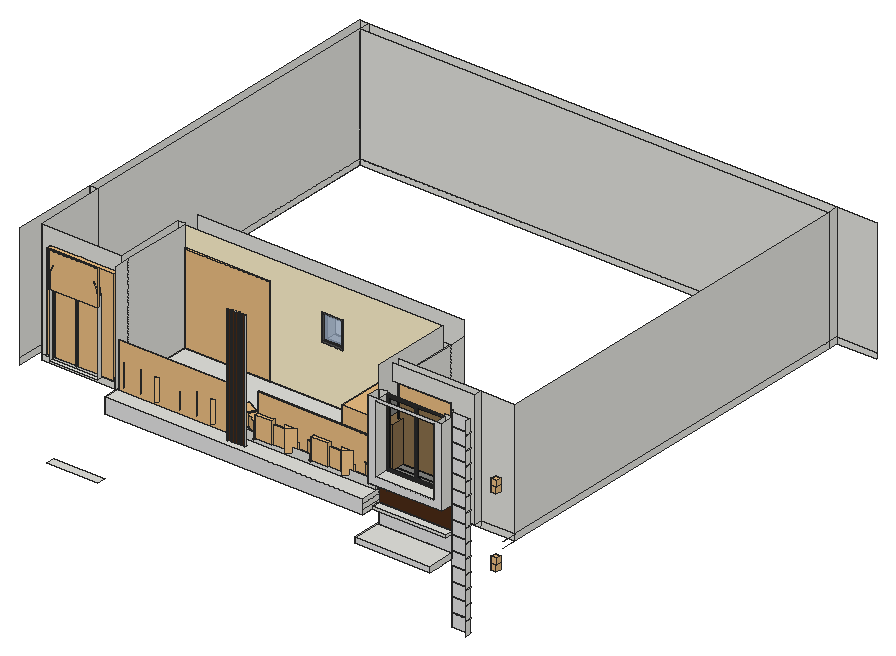
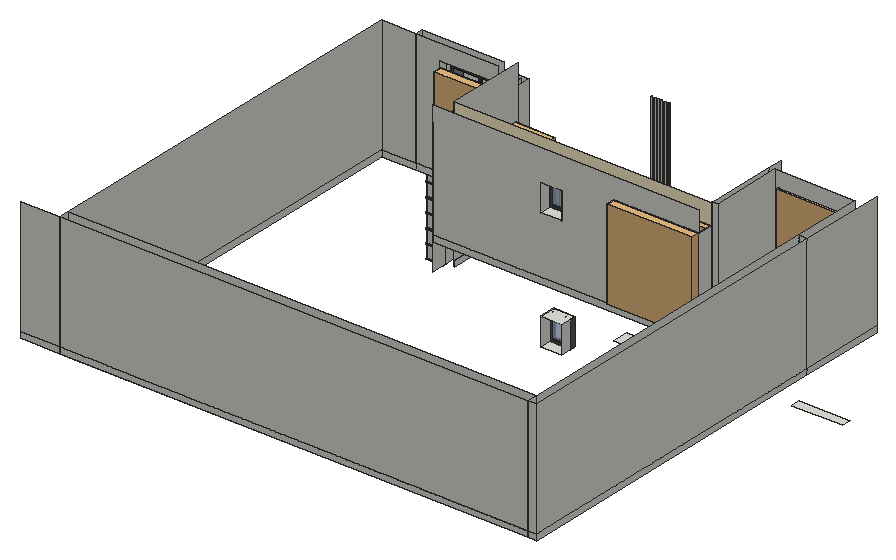
# SketchUp Ruby script. Lengths in inches.
U = 1.inch
M = Sketchup.active_model
def pt(a) = Geom::Point3d.new(a.map { |v| v * U })
def face(e, loops, mat)
  f = e.add_face(loops[0].map { |a| pt(a) })
  loops[1..].each { |l| e.add_face(l.map { |a| pt(a) }).erase! }
  f.material = f.back_material = mat if mat
  f
end
# faces: each face lists its corners as indices into pts; further lists are holes
def faces(e, pts, list, mat = nil) = list.each { |f| face(e, (f[0].is_a?(Array) ? f : [f]).map { |l| l.map { |i| pts[i] } }, mat) }
# xy, xz, yz: faces in a plane at the given z, y or x. An outline is a flat list of corners, or four numbers for a rectangle; further outlines are holes
def ring(l) = l.size == 4 ? [[l[0], l[1]], [l[2], l[1]], [l[2], l[3]], [l[0], l[3]]] : l.each_slice(2).to_a
def flat(e, list, mat, &to3) = list.each { |f| face(e, (f[0].is_a?(Array) ? f : [f]).map { |l| ring(l).map { |u, v| to3.(u, v) } }, mat) }
def xy(e, z, list, mat = nil) = flat(e, list, mat) { |x, y| [x, y, z] }
def xz(e, y, list, mat = nil) = flat(e, list, mat) { |x, z| [x, y, z] }
def yz(e, x, list, mat = nil) = flat(e, list, mat) { |y, z| [x, y, z] }
def lines(e, pts, list) = list.each { |a, b| e.add_line(pt(pts[a]), pt(pts[b])) }
# prism: a flat outline (further loops are holes) pulled along v
def prism(e, loops, v, mat = nil)
  f = face(e, loops, mat); d = Geom::Vector3d.new(v.map { |x| x * U })
  f.pushpull(f.normal.samedirection?(d) ? d.length : -d.length)
end
def box(e, o, s, mat = nil) = prism(e, [[o, [o[0] + s[0], o[1], o[2]], [o[0] + s[0], o[1] + s[1], o[2]], [o[0], o[1] + s[1], o[2]]]], [0, 0, s[2]], mat)
def at(x, y, z, deg = 0) = Geom::Transformation.translation(pt([x, y, z])) * Geom::Transformation.rotation(ORIGIN, Z_AXIS, deg.degrees)
def axes(o, x, y, z) = Geom::Transformation.new([*x, 0, *y, 0, *z, 0, *pt(o).to_a, 1])
def part(name) = M.definitions.add(name)
# library, detail: a bought-in or finely detailed component or shape, given as its bounding box
def library(name, o, s) = part(name).tap { |d| box(d.entities, o, s) }
def detail(e, o, s) = box(e.add_group.entities, o, s)
def put(e, d, t, mat = nil) = e.add_instance(d, t).tap { |i| i.material = mat if mat }
def group(e, t, mat = nil) = e.add_group.tap { |g| g.transformation = t; g.material = mat if mat }.entities
root = M.entities
M.materials.add("Glass_Tinted_Gray").color = [0, 0, 0]
M.materials["Glass_Tinted_Gray"].alpha = 0.125
M.materials.add("Material__1").color = [95, 70, 46]
M.materials.add("[0135_DarkGray]").color = [81, 81, 81]
M.materials.add("[Color D01]").color = [255, 242, 204]
M.materials.add("[Color M01]").color = [226, 226, 226]
M.materials.add("[Color_006]").color = [86, 86, 86]
M.materials.add("[Mirror 02]").color = [229, 229, 229]
M.materials.add("[Terrazzo Light Blue]").color = [196, 214, 227]
M.materials.add("[Translucent Glass Gray]").color = [128, 128, 128]
M.materials["[Translucent Glass Gray]"].alpha = 0.5
M.materials.add("[Translucent_Glass_Gray]1").color = [167, 187, 214]
M.materials["[Translucent_Glass_Gray]1"].alpha = 0.8
M.materials.add("[Wood Veneer 01]").color = [76, 44, 23]
c1 = part("BIC_Bike Shop - Window - Small")
xy(c1.entities,-8,[[[0,0,36,36],[2,2,34,34]]],"[Color_006]")
xy(c1.entities,-4,[[2,2,34,34]],"[Translucent_Glass_Gray]1")
xy(c1.entities,0,[[[0,0,36,36],[2,2,34,34]]],"[Color_006]")
xz(c1.entities,0,[[0,-8,36,0]],"[Color_006]")
xz(c1.entities,2,[[2,-8,34,-4],[2,-4,34,0]],"[Color_006]")
xz(c1.entities,34,[[2,-8,34,-4],[2,-4,34,0]],"[Color_006]")
xz(c1.entities,36,[[0,-8,36,0]],"[Color_006]")
yz(c1.entities,0,[[0,-8,36,0]],"[Color_006]")
yz(c1.entities,2,[[2,-8,34,-4],[2,-4,34,0]],"[Color_006]")
yz(c1.entities,34,[[2,-8,34,-4],[2,-4,34,0]],"[Color_006]")
yz(c1.entities,36,[[0,-8,36,0]],"[Color_006]")
c2 = library("SPOT",[0,0,1.68],[5.4375,5.4375,6.28])
c3 = part("Group\#3")
xy(c3.entities,0,[[0,0,32.48,1.97]])
xy(c3.entities,0.98,[[0.98,0,31.5,0.98],[0.98,0.98,31.5,1.97]])
xy(c3.entities,8.86,[[0.98,0,31.5,0.98],[0.98,0.98,31.5,1.97]])
xy(c3.entities,9.84,[[0,0,32.48,1.97]])
xz(c3.entities,0,[[[0,0,32.48,9.84],[0.98,0.98,31.5,8.86]]])
xz(c3.entities,0.98,[[0.98,0.98,31.5,8.86]],"[Translucent Glass Gray]")
xz(c3.entities,1.97,[[[0,0,32.48,9.84],[0.98,0.98,31.5,8.86]]])
yz(c3.entities,0,[[0,0,1.97,9.84]])
yz(c3.entities,0.98,[[0,0.98,0.98,8.86],[0.98,0.98,1.97,8.86]])
yz(c3.entities,31.5,[[0,0.98,0.98,8.86],[0.98,0.98,1.97,8.86]])
yz(c3.entities,32.48,[[0,0,1.97,9.84]])
c4 = part("Group\#4")
xy(c4.entities,0,[[0,0,32.48,1.97]])
xy(c4.entities,0.98,[[0.98,0,31.5,0.98],[0.98,0.98,31.5,1.97]])
xy(c4.entities,71.85,[[0.98,0,31.5,0.98],[0.98,0.98,31.5,1.97]])
xy(c4.entities,72.83,[[0,0,32.48,1.97]])
xz(c4.entities,0,[[[0,0,32.48,72.83],[0.98,0.98,31.5,71.85]]])
xz(c4.entities,0.98,[[0.98,0.98,31.5,71.85]],"[Translucent Glass Gray]")
xz(c4.entities,1.97,[[[0,0,32.48,72.83],[0.98,0.98,31.5,71.85]]])
yz(c4.entities,0,[[0,0,1.97,72.83]])
yz(c4.entities,0.98,[[0,0.98,0.98,71.85],[0.98,0.98,1.97,71.85]])
yz(c4.entities,31.5,[[0,0.98,0.98,71.85],[0.98,0.98,1.97,71.85]])
yz(c4.entities,32.48,[[0,0,1.97,72.83]])
c5 = part("FIXED+GLASS+WINDOW+WITH+TRANSOM")
g1 = group(c5.entities,at(0,0,0))
xy(g1,0,[[0,0,70.86,3.9375]])
xy(g1,1.97,[[1.97,0,34.45,0.98],[36.42,0,68.9,3.9375],[1.97,2.95,34.45,3.9375]])
xy(g1,86.61,[[1.97,0,34.45,3.9375],[34.45,0,36.42,3.9375],[36.42,0,68.9,3.9375]])
xy(g1,88.58,[[0,0,70.86,3.9375]])
xz(g1,0,[[[0,0,70.86,88.58],[1.97,1.97,34.45,86.61],[36.42,1.97,68.9,86.61]]])
xz(g1,3.9375,[[[0,0,70.86,88.58],[1.97,1.97,34.45,86.61],[36.42,1.97,68.9,86.61]]])
yz(g1,0,[[0,0,3.9375,88.58]])
yz(g1,1.97,[[0,1.97,3.9375,74.8],[0,76.77,3.9375,86.61]])
yz(g1,34.45,[[0,1.97,3.9375,86.61]])
yz(g1,36.42,[[0,1.97,3.9375,86.61]])
yz(g1,68.9,[[0,1.97,3.9375,86.61]])
yz(g1,70.86,[[0,0,3.9375,88.58]])
g2 = group(g1,at(1.97,0,74.8))
box(g2,[0,0,0],[66.93,3.9375,1.97])
put(g1,c3,at(1.97,0.98,76.77))
put(g1,c3,at(36.42,0.98,76.77))
put(g1,c4,at(1.97,0.98,1.97))
put(g1,c4,at(36.42,0.98,1.97))
c6 = library("Sliding Door",[0,0,0],[94.49,5.83,91.73])
c7 = library("Flora+17",[-57.52,158.6,-38.64],[66.99,62.88,77.28])
c8 = part("glass-railing")
detail(c8.entities,[0,0,0],[1.26,75.59,33.1875])
c9 = library("Areca palm plant",[0,0,0],[49.1,36.6,54.46])
c10 = library("Group20\#1",[-20.81,-17.08,3.79],[39.86,39.43,37.51])
c11 = library("Group\#74",[-84.69,-90.07,-0.36],[176.51,175.13,171.4])
c12 = library("Group\#130",[-7.34,-1.2,0],[38.67,35.81,49.04])
c13 = library("Group38\#2",[14.01,28.44,-23.43],[18.58,18.32,38.89])
c14 = part("Group\#11")
put(c14.entities,c9,axes([-6.2,56.6,6.08],[0.45017,-0.56191,0],[0.66137,0.52986,0],[0,0,0.72]))
put(c14.entities,c9,axes([-6.2,158.41,6.08],[0.45017,-0.56191,0],[0.66137,0.52986,0],[0,0,0.72]))
put(c14.entities,c10,axes([18.97,181.79,4.77],[0,0.85,0],[-0.85,0,0],[0,0,0.85]))
put(c14.entities,c11,axes([14.93,71.3,6.05],[-0.04961,-0.08593,0],[0.08593,-0.04961,0],[0,0,0.10522]))
put(c14.entities,c11,axes([14.93,91.37,6.05],[-0.04961,-0.08593,0],[0.08593,-0.04961,0],[0,0,0.10522]))
put(c14.entities,c10,axes([18.97,79.98,4.77],[0,0.85,0],[-0.85,0,0],[0,0,0.85]))
put(c14.entities,c12,axes([24.9375,191.72,8],[0,0.79,0],[-0.79,0,0],[0,0,0.79]))
put(c14.entities,c11,axes([17.19,223.04,6.07],[-0.08133,-0.14087,0],[0.14087,-0.08133,0],[0,0,0.1725]))
put(c14.entities,c12,axes([24.9375,89.91,8],[0,0.79,0],[-0.79,0,0],[0,0,0.79]))
put(c14.entities,c11,axes([14.93,44.05,6.05],[-0.04961,-0.08593,0],[0.08593,-0.04961,0],[0,0,0.10522]))
put(c14.entities,c11,axes([14.93,145.87,6.05],[-0.04961,-0.08593,0],[0.08593,-0.04961,0],[0,0,0.10522]))
put(c14.entities,c13,axes([-4.1,100.66,28.17],[0.8848,0,0],[0,0.94674,0],[0,0,0.85826]))
put(c14.entities,c11,axes([14.93,173.12,6.05],[-0.04961,-0.08593,0],[0.08593,-0.04961,0],[0,0,0.10522]))
put(c14.entities,c13,axes([-4.1,-1.15,28.17],[0.8848,0,0],[0,0.94674,0],[0,0,0.85826]))
put(c14.entities,c11,axes([17.19,121.23,6.07],[-0.08133,-0.14087,0],[0.14087,-0.08133,0],[0,0,0.1725]))
put(c14.entities,c11,axes([14.93,193.18,6.05],[-0.04961,-0.08593,0],[0.08593,-0.04961,0],[0,0,0.10522]))
put(c14.entities,c11,axes([17.19,15.79,6.07],[-0.08133,-0.14087,0],[0.14087,-0.08133,0],[0,0,0.1725]))
g3 = group(c14.entities,at(0,0,0))
xy(g3,0,[[0,0,6,234.8],[30,0,36,234.8]])
xy(g3,3,[[6,0,30,234.8]])
xy(g3,7,[[6,5,30,229.8]],"Material__1")
xy(g3,15,[[[0,0,36,234.8],[6,5,30,229.8]]])
xz(g3,0,[[0,0,6,0,6,3,30,3,30,0,36,0,36,15,0,15]])
xz(g3,5,[[6,7,30,15]])
xz(g3,229.8,[[6,7,30,15]])
xz(g3,234.8,[[0,0,0,15,36,15,36,0,30,0,30,3,6,3,6,0]])
yz(g3,0,[[0,0,234.8,15]])
yz(g3,6,[[0,0,234.8,3],[5,7,229.8,15]])
yz(g3,30,[[0,0,234.8,3],[5,7,229.8,15]])
yz(g3,36,[[0,0,234.8,15]])
c15 = library("Curtains",[0,0,0],[121.73,8.19,117.22])
c16 = part("PENTEK_RP Fineline 50S_Sliding_DoorCase_E1")
box(c16.entities,[0,0,0],[1.51,3.66,99.27],"[0135_DarkGray]")
c17 = part("PENTEK_RP Fineline 50S_SlidingDooe_Case_E2")
box(c17.entities,[0,0,0],[96.25,3.66,1.51],"[0135_DarkGray]")
c18 = part("pentek_RP Fineline 50S_SlidingDoor_Case")
put(c18.entities,c16,at(97.76,0,0))
put(c18.entities,c17,at(1.51,0,0))
put(c18.entities,c16,at(0,0,0))
put(c18.entities,c17,at(1.51,0,97.76))
c19 = part("PENTEK_RP Fineline 50S_SlidingDoor_GlazingBead_2")
box(c19.entities,[0,0,0],[0.56,0.59,94.39],"[0135_DarkGray]")
c20 = part("PENTEK_RP Fineline 50S_SlidingDoor_Glass")
box(c20.entities,[0,0,0],[46.58,0.16,94.39],"Glass_Tinted_Gray")
c21 = part("PENTEK_RP Fineline 50S_SlidingDoor_GlazingBead")
box(c21.entities,[0,0,0],[45.47,0.59,0.56],"[0135_DarkGray]")
c22 = part("PENTEK_RP Fineline 50S_SlidingDoor_Leaf_E1")
xy(c22.entities,0,[[0,0,0.93,1.97],[0.93,1.57,1.49,1.97]],"[0135_DarkGray]")
xy(c22.entities,96.25,[[0,0,0.93,0,0.93,1.57,1.49,1.57,1.49,1.97,0,1.97]],"[0135_DarkGray]")
xz(c22.entities,0,[[0,0,0.93,96.25]],"[0135_DarkGray]")
xz(c22.entities,1.57,[[0.93,0,1.49,95.32],[0.93,95.32,1.49,96.25]],"[0135_DarkGray]")
xz(c22.entities,1.97,[[0,0,1.49,96.25]],"[0135_DarkGray]")
yz(c22.entities,0,[[0,0,1.97,96.25]],"[0135_DarkGray]")
yz(c22.entities,0.93,[[0,0,1.57,0.93],[0,0.93,1.57,95.32],[0,95.32,1.57,96.25]],"[0135_DarkGray]")
yz(c22.entities,1.49,[[1.57,0,1.97,95.32],[1.57,95.32,1.97,96.25]],"[0135_DarkGray]")
c23 = part("PENTEK_RP Fineline 50S_SlidingDoor_Leaf_E2")
xy(c23.entities,0,[[0,0,0,1.57,0.56,1.57,0.56,1.97,46.02,1.97,46.02,1.57,46.58,1.57,46.58,0]],"[0135_DarkGray]")
xy(c23.entities,0.93,[[0,0,46.58,1.57]],"[0135_DarkGray]")
xy(c23.entities,1.49,[[0.56,1.57,46.02,1.97]],"[0135_DarkGray]")
xz(c23.entities,0,[[0,0,46.58,0.93]],"[0135_DarkGray]")
xz(c23.entities,1.57,[[0,0,0.56,0.93],[46.02,0,46.58,0.93],[0.56,0.93,46.02,1.49]],"[0135_DarkGray]")
xz(c23.entities,1.97,[[0.56,0,46.02,1.49]],"[0135_DarkGray]")
yz(c23.entities,0,[[0,0,1.57,0.93]],"[0135_DarkGray]")
yz(c23.entities,0.56,[[1.57,0,1.97,0.93],[1.57,0.93,1.97,1.49]],"[0135_DarkGray]")
yz(c23.entities,46.02,[[1.57,0,1.97,0.93],[1.57,0.93,1.97,1.49]],"[0135_DarkGray]")
yz(c23.entities,46.58,[[0,0,1.57,0.93]],"[0135_DarkGray]")
c24 = part("PENTEK_RP Fineline S_SlidingDoor_Leaf1")
put(c24.entities,c19,at(0.93,0,0.93))
put(c24.entities,c19,at(46.96,0,0.93))
put(c24.entities,c20,at(1.49,1.42,0.93))
put(c24.entities,c21,at(1.49,0,0.93))
put(c24.entities,c20,at(1.49,0.59,0.93),"[Terrazzo Light Blue]")
put(c24.entities,c22,at(0,0,0))
put(c24.entities,c22,axes([48.44,0,0],[-1,0,0],[0,1,0],[0,0,1]))
put(c24.entities,c23,axes([0.93,0,96.25],[1,0,0],[0,1,0],[0,0,-1]))
put(c24.entities,c23,at(0.93,0,0))
put(c24.entities,c21,at(1.49,0,94.77))
c25 = part("PENTEK_RP Fineline 50S_SlidingDoor_Leaf2")
put(c25.entities,c20,at(1.49,1.42,0.93))
put(c25.entities,c21,at(1.49,0,94.77))
put(c25.entities,c19,at(46.96,0,0.93))
put(c25.entities,c20,at(1.49,0.59,0.93),"[Mirror 02]")
put(c25.entities,c19,at(0.93,0,0.93))
put(c25.entities,c22,at(0,0,0))
put(c25.entities,c22,axes([48.44,0,0],[-1,0,0],[0,1,0],[0,0,1]))
put(c25.entities,c21,at(1.49,0,0.93))
put(c25.entities,c23,axes([0.93,0,96.25],[1,0,0],[0,1,0],[0,0,-1]))
put(c25.entities,c23,at(0.93,0,0))
c26 = part("PENTEK - Slimmest Steel Sliding Door / Window\#1")
put(c26.entities,c18,at(0,-1.88,-0.09))
put(c26.entities,c24,at(1.51,-2.27,1.42))
put(c26.entities,c25,at(49.32,-0.3,1.42))
c27 = library("Group\#1",[0,0,0],[33.46,1.57,19.69])
xy(root,167.92,[[733.09,261.68,751.93,263.24]])
xy(root,171.49,[[314.4,263.24,366.4,272.46]])
xy(root,181.28,[[733.09,261.68,751.93,263.24]])
xy(root,182.22,[[733.09,261.68,751.93,263.24]])
xy(root,195.58,[[733.09,261.68,751.93,263.24]])
xy(root,196.52,[[733.09,261.68,751.93,263.24]])
xy(root,199.5625,[[531.79,345.71,553.72,362.65]])
xy(root,209.875,[[733.09,261.68,751.93,263.24]])
xy(root,210.8125,[[733.09,261.68,751.93,263.24]])
xy(root,224.18,[[733.09,261.68,751.93,263.24]])
xy(root,225.11,[[733.09,261.68,751.93,263.24]])
xy(root,227.9375,[[531.79,345.71,553.72,362.65]])
xy(root,229.87,[[664.71,249.36,724.59,279.2],[664.71,279.2,665.11,345.71],[665.11,279.2,665.59,345.71]])
xy(root,229.99,[[[655.52,234.3,732.65,249.36],[693.1875,238.33,693.82,238.42,694.41,238.66,694.91,239.05,695.3,239.55,695.54,240.14,695.625,240.77,695.54,241.4,695.3,241.99,694.91,242.49,694.41,242.88,693.82,243.125,693.1875,243.21,692.56,243.125,691.97,242.88,691.46,242.49,691.08,241.99,690.83,241.4,690.75,240.77,690.83,240.14,691.08,239.55,691.46,239.05,691.97,238.66,692.56,238.42]]])
xy(root,230.43,[[655.52,249.36,657.09,345.71],[657.09,249.36,732.65,263.24],[732.65,249.36,733.09,263.24]])
xy(root,230.62,[[693.1875,238.33,692.56,238.42,691.97,238.66,691.46,239.05,691.08,239.55,690.83,240.14,690.75,240.77,690.83,241.4,691.08,241.99,691.46,242.49,691.97,242.88,692.56,243.125,693.1875,243.21,693.82,243.125,694.41,242.88,694.91,242.49,695.3,241.99,695.54,241.4,695.625,240.77,695.54,240.14,695.3,239.55,694.91,239.05,694.41,238.66,693.82,238.42]])
xy(root,231.125,[[390.34,345.71,390.9,362.65],[390.9,345.71,478.4,362.65]])
xy(root,235.64,[[655.52,234.3,732.65,234.3,732.65,263.24,657.09,263.24,657.09,345.71,655.52,345.71]])
xy(root,238.47,[[733.09,261.68,751.93,263.24]])
xy(root,239.41,[[733.09,261.68,751.93,263.24]])
xy(root,252.77,[[733.09,261.68,751.93,263.24]])
xy(root,253.375,[[657.09,254.43,733.09,263.24]])
xy(root,253.375,[[[390.34,242.18,657.09,345.71],[447.91,289.875,449.21,289.96,450.45,290.37,451.53,291.09,452.4,292.07,452.98,293.24,453.24,294.52,453.16,295.82,452.75,297.06,452.03,298.14,451.05,299.01,449.88,299.59,448.6,299.85,447.3,299.77,446.0625,299.36,444.97,298.64,444.11,297.66,443.53,296.49,443.27,295.21,443.35,293.91,443.76,292.67,444.48,291.58,445.46,290.72,446.625,290.14],[595.53,289.875,596.83,289.96,598.07,290.37,599.16,291.09,600.02,292.07,600.61,293.24,600.87,294.52,600.79,295.82,600.37,297.06,599.65,298.14,598.67,299.01,597.51,299.59,596.23,299.85,594.92,299.77,593.6875,299.36,592.6,298.64,591.73,297.66,591.15,296.49,590.89,295.21,590.97,293.91,591.39,292.67,592.11,291.58,593.08,290.72,594.25,290.14]]],"[Wood Veneer 01]")
xy(root,253.71,[[733.09,261.68,751.93,263.24]])
xy(root,254.4375,[[447.91,289.875,446.625,290.14,445.46,290.72,444.48,291.58,443.76,292.67,443.35,293.91,443.27,295.21,443.53,296.49,444.11,297.66,444.97,298.64,446.0625,299.36,447.3,299.77,448.6,299.85,449.88,299.59,451.05,299.01,452.03,298.14,452.75,297.06,453.16,295.82,453.24,294.52,452.98,293.24,452.4,292.07,451.53,291.09,450.45,290.37,449.21,289.96],[595.53,289.875,594.25,290.14,593.08,290.72,592.11,291.58,591.39,292.67,590.97,293.91,590.89,295.21,591.15,296.49,591.73,297.66,592.6,298.64,593.6875,299.36,594.92,299.77,596.23,299.85,597.51,299.59,598.67,299.01,599.65,298.14,600.37,297.06,600.79,295.82,600.87,294.52,600.61,293.24,600.02,292.07,599.16,291.09,598.07,290.37,596.83,289.96]])
xy(root,255.91,[[657.09,254.43,733.09,263.24]])
xy(root,258,[[292.06,345.71,301.28,694.43],[301.28,683.75,784.56,694.43]])
xy(root,259.25,[[511.65,248.63,512.53,250.63],[529.78,248.63,530.65,250.63],[526.41,249.32,529.24,250.63],[512.53,249.76,515.36,250.63],[516,249.76,518.83,250.63],
  [519.47,249.76,522.3,250.63],[522.9375,249.76,525.77,250.63]])
xy(root,264,[[665.11,271.58,749.59,279.2],[292.06,345.71,301.28,694.43],[301.28,683.75,784.56,694.43]])
xy(root,267.07,[[733.09,261.68,751.93,263.24]])
xy(root,267.28,[[316.75,263.24,366.25,272.46]])
xy(root,268.01,[[733.09,261.68,751.93,263.24]])
xy(root,268.625,[[390.34,242.18,657.09,345.71],[511.65,248.63,512.53,250.63],[529.78,248.63,530.65,250.63],[512.53,249.32,515.36,250.63],[516,249.32,518.83,250.63],
  [519.47,249.32,522.3,250.63],[522.9375,249.32,525.77,250.63],[526.41,249.32,529.24,250.63],[390.34,345.71,390.9,362.65],[390.9,345.71,478.4,362.65]])
xy(root,280.21,[[657.09,249.36,732.9,263.24]])
xy(root,281.37,[[733.09,261.68,751.93,263.24]])
xy(root,282.31,[[733.09,261.68,751.93,263.24]])
xy(root,288.24,[[664.71,249.36,724.59,263.24],[664.71,263.24,724.59,263.24,724.59,271.58,665.11,271.58,665.11,279.2,664.71,279.2],[665.11,271.58,724.59,279.2]])
xy(root,292.81,[[664.05,279.2,665.11,345.71]])
xy(root,295.67,[[733.09,261.68,751.93,263.24]])
xy(root,296.61,[[733.09,261.68,751.93,263.24]])
xy(root,309.97,[[733.09,261.68,751.93,263.24]])
xy(root,310.91,[[733.09,261.68,751.93,263.24]])
xy(root,323.625,[[531.79,345.71,553.72,362.65]])
xy(root,324.27,[[733.09,261.68,751.93,263.24]])
xy(root,325.2,[[733.09,261.68,751.93,263.24]])
xy(root,338.57,[[733.09,261.68,751.93,263.24]])
xy(root,339.5,[[733.09,261.68,751.93,263.24]])
xy(root,352,[[531.79,345.71,553.72,362.65]])
xy(root,352.86,[[733.09,261.68,751.93,263.24]])
xy(root,353.8,[[733.09,261.68,751.93,263.24]])
xz(root,234.3,[[655.52,229.99,732.65,235.64]],"[Color M01]")
xz(root,242.18,[[390.34,253.375,657.09,268.625]],"[Color M01]")
xz(root,248.63,[[511.65,268.625,512.53,389.875],[529.78,268.625,530.65,389.875]])
xz(root,249.32,[[512.53,268.625,515.36,389.875],[516,268.625,518.83,389.875],[519.47,268.625,522.3,389.875],[522.9375,268.625,525.77,389.875],[526.41,268.625,529.24,389.875]],"[Wood Veneer 01]")
xz(root,249.36,[[655.52,229.99,657.09,230.43],[657.09,229.99,732.65,230.43]])
xz(root,249.36,[[[657.09,280.21,732.9,361.12],[664.71,288.24,724.59,358.37]]],"[Color M01]")
xz(root,254.43,[[657.09,253.375,733.09,255.91]])
xz(root,261.68,[[733.09,296.61,751.93,309.97]])
xz(root,261.68,[[733.09,167.92,751.93,181.28],[733.09,182.22,751.93,195.58],[733.09,196.52,751.93,209.875],[733.09,210.8125,751.93,224.18],[733.09,225.11,751.93,238.47],
  [733.09,239.41,751.93,252.77],[733.09,253.71,751.93,267.07],[733.09,268.01,751.93,281.37],[733.09,282.31,751.93,295.67],[733.09,310.91,751.93,324.27],
  [733.09,325.2,751.93,338.57],[733.09,339.5,751.93,352.86],[733.09,353.8,751.93,367.16]],"[Color M01]")
xz(root,263.24,[[733.09,181.28,751.93,182.22],[733.09,195.58,751.93,196.52],[733.09,209.875,751.93,210.8125],[733.09,224.18,751.93,225.11],[657.09,230.43,732.65,235.64],
  [733.09,238.47,751.93,239.41],[733.09,252.77,751.93,253.71],[657.09,253.375,733.09,255.91],[733.09,267.07,751.93,268.01],[657.09,280.21,664.71,361.12],
  [664.71,280.21,664.71,288.24,724.59,288.24,724.59,361.12,732.9,361.12,732.9,280.21],[733.09,281.37,751.93,282.31],[733.09,295.67,751.93,296.61],[733.09,309.97,751.93,310.91],[733.09,324.27,751.93,325.2],
  [733.09,338.57,751.93,339.5],[733.09,352.86,751.93,353.8]])
xz(root,263.24,[[732.65,230.43,733.09,230.43,733.09,253.375,657.09,253.375,657.09,235.64,732.65,235.64]],"[Color M01]")
xz(root,263.24,[[657.09,255.91,733.09,255.91,733.09,367.82,732.9,367.82,732.9,280.21,657.09,280.21]],"[Wood Veneer 01]")
xz(root,271.58,[[665.11,264,749.59,264,749.59,384,665.11,384,665.11,367.49,724.59,367.49,724.59,288.24,665.11,288.24]])
xz(root,272.46,[[301.28,258,383.72,264],[[301.28,264,383.72,384],[316.75,267.28,366.25,267.28,366.25,343.59,365.41,350,362.9375,355.97,359,361.09,353.875,365.03,347.91,367.5,341.5,368.34,335.1,367.5,329.125,365.03,324,361.09,320.07,355.97,317.6,350,316.75,343.59]]])
xz(root,279.2,[[665.11,258,749.59,264],[749.59,258,784.56,264],[665.11,264,665.11,288.24,724.59,288.24,724.59,367.49,665.11,367.49,665.11,384,749.59,384,749.59,264],[749.59,264,784.56,384],[664.71,288.24,665.11,292.81],
  [664.05,292.81,664.71,367.49],[664.71,292.81,665.11,367.49]])
xz(root,345.71,[[390.34,253.375,657.09,258],[292.06,258,301.28,264],[383.72,258,390.34,264],[292.06,264,301.28,384],[383.72,264,390.34,384],
  [390.34,264,657.09,268.625],[390.34,268.625,390.9,361.75],[657.09,268.625,657.09,367.82,664.71,367.82,664.71,367.49,664.05,367.49,664.05,292.81,664.71,292.81,664.71,268.625],[664.05,292.81,664.71,367.49],[664.71,292.81,665.11,367.49]])
xz(root,345.71,[[[478.4,268.625,657.09,268.625,657.09,382.6875,390.34,382.6875,390.34,361.75,478.4,361.75],[531.79,323.625,553.72,352]]],"[Color D01]")
xz(root,362.65,[[390.34,258,665.11,264],[[390.34,264,390.34,268.625,478.4,268.625,478.4,361.75,390.34,361.75,390.34,384,665.11,384,665.11,264],[531.79,323.625,553.72,352]],[390.34,268.625,390.9,361.75]])
xz(root,683.75,[[301.28,258,784.56,264],[301.28,264,784.56,384]])
xz(root,694.43,[[292.06,258,301.28,264],[301.28,258,784.56,264],[784.56,258,825.43,264],[292.06,264,301.28,384],[301.28,264,784.56,384],
  [784.56,264,825.43,384]])
yz(root,292.06,[[256.61,258,345.71,264],[345.71,258,694.43,264],[256.61,264,345.71,384],[345.71,264,694.43,384]])
yz(root,301.28,[[272.46,258,345.71,264],[345.71,258,683.75,264],[683.75,258,694.43,264],[272.46,264,345.71,384],[345.71,264,683.75,384],
  [683.75,264,694.43,384]])
yz(root,316.75,[[263.24,267.28,272.46,343.59]])
yz(root,366.25,[[263.24,267.28,272.46,343.59]])
yz(root,383.72,[[272.46,258,345.71,264],[272.46,264,345.71,384]])
yz(root,390.34,[[345.71,231.125,362.65,258],[242.18,253.375,256.61,258],[256.61,253.375,272.46,258],[272.46,253.375,345.71,258],[242.18,258,256.61,264],
  [256.61,258,272.46,264],[272.46,258,345.71,264],[345.71,258,362.65,264],[242.18,264,256.61,268.625],[256.61,264,272.46,268.625],
  [272.46,264,345.71,268.625],[345.71,264,362.65,268.625],[256.61,268.625,272.46,382.6875],[272.46,268.625,345.71,382.6875],[345.71,268.625,362.65,361.75]])
yz(root,390.9,[[345.71,268.625,362.65,361.75]])
yz(root,478.4,[[345.71,268.625,362.65,361.75]])
yz(root,512.53,[[248.63,268.625,249.32,389.875]])
yz(root,515.36,[[249.32,268.625,250.63,389.875]])
yz(root,516,[[249.32,268.625,250.63,389.875]])
yz(root,518.83,[[249.32,268.625,250.63,389.875]])
yz(root,519.47,[[249.32,268.625,250.63,389.875]])
yz(root,522.3,[[249.32,268.625,250.63,389.875]])
yz(root,522.9375,[[249.32,268.625,250.63,389.875]])
yz(root,525.77,[[249.32,268.625,250.63,389.875]])
yz(root,526.41,[[249.32,268.625,250.63,389.875]])
yz(root,529.24,[[249.32,268.625,250.63,389.875]])
yz(root,529.78,[[248.63,268.625,250.63,389.875]])
yz(root,531.79,[[345.71,199.5625,362.65,227.9375],[345.71,323.625,362.65,352]])
yz(root,553.72,[[345.71,199.5625,362.65,227.9375],[345.71,323.625,362.65,352]])
yz(root,655.52,[[234.3,229.99,234.3,235.64,345.71,235.64,345.71,230.43,249.36,230.43,249.36,229.99]])
yz(root,657.09,[[263.24,230.43,345.71,235.64],[263.24,235.64,345.71,253.375],[242.18,253.375,254.43,253.375,254.43,255.91,259.36,255.91,259.36,258,242.18,258],[254.43,253.375,263.24,255.91],[263.24,253.375,345.71,258],
  [259.36,255.91,263.24,258],[242.18,258,263.24,264],[242.18,264,263.24,268.625],[263.24,264,345.71,268.625],[263.24,268.625,345.71,382.6875],
  [249.36,280.21,263.24,361.12]])
yz(root,664.05,[[279.2,292.81,345.71,367.49]])
yz(root,664.71,[[249.36,288.24,263.24,358.37]])
yz(root,665.11,[[279.2,229.87,345.71,258],[345.71,229.87,362.65,258],[279.2,258,345.71,264],[345.71,258,362.65,264],[271.58,264,279.2,288.24],
  [279.2,264,345.71,292.81],[345.71,264,362.65,292.81],[279.2,292.81,345.71,367.49],[345.71,292.81,362.65,367.49]])
yz(root,724.59,[[249.36,288.24,263.24,358.37],[271.58,288.24,279.2,367.49]])
yz(root,732.65,[[234.3,229.99,249.36,229.99,249.36,230.43,263.24,230.43,263.24,235.64,234.3,235.64]])
yz(root,732.9,[[249.36,280.21,263.24,361.12]])
yz(root,733.09,[[261.68,167.92,263.24,181.28],[261.68,182.22,263.24,195.58],[261.68,196.52,263.24,209.875],[261.68,210.8125,263.24,224.18],[261.68,230.43,263.24,238.47],
  [261.68,239.41,263.24,252.77],[254.43,253.375,263.24,253.375,263.24,253.71,261.68,253.71,261.68,255.91,254.43,255.91],[261.68,253.71,263.24,255.91],[261.68,255.91,263.24,267.07],[261.68,268.01,263.24,281.37],
  [261.68,282.31,263.24,295.67],[261.68,296.61,263.24,309.97],[261.68,310.91,263.24,324.27],[261.68,325.2,263.24,338.57],[261.68,339.5,263.24,352.86],
  [261.68,353.8,263.24,367.16]])
yz(root,749.59,[[271.58,264,279.2,384]])
yz(root,751.93,[[256.61,167.92,261.68,181.28],[256.61,181.28,263.24,182.22],[256.61,182.22,261.68,195.58],[256.61,195.58,263.24,196.52],[256.61,196.52,261.68,209.875],
  [256.61,209.875,263.24,210.8125],[256.61,210.8125,261.68,224.18],[256.61,224.18,263.24,225.11],[256.61,225.11,261.68,238.47],[256.61,238.47,263.24,239.41],
  [256.61,239.41,261.68,252.77],[256.61,252.77,263.24,253.71],[256.61,253.71,261.68,267.07],[256.61,267.07,263.24,268.01],[256.61,268.01,261.68,281.37],
  [256.61,281.37,263.24,282.31],[256.61,282.31,261.68,295.67],[256.61,295.67,263.24,296.61],[256.61,296.61,261.68,309.97],[256.61,309.97,263.24,310.91],
  [256.61,310.91,261.68,324.27],[256.61,324.27,263.24,325.2],[256.61,325.2,261.68,338.57],[256.61,338.57,263.24,339.5],[256.61,339.5,261.68,352.86],
  [256.61,352.86,263.24,353.8],[256.61,353.8,261.68,367.16]])
yz(root,784.56,[[279.2,258,683.75,264],[683.75,258,694.43,264],[279.2,264,683.75,384],[683.75,264,694.43,384]])
p = [[693.1875,238.33,229.99],[692.56,238.42,229.99],[692.56,238.42,230.62],[693.1875,238.33,230.62],[693.82,238.42,229.99],[693.82,238.42,230.62],
  [691.97,238.66,229.99],[691.97,238.66,230.62],[694.41,238.66,229.99],[694.41,238.66,230.62],[691.46,239.05,229.99],[691.46,239.05,230.62],
  [694.91,239.05,229.99],[694.91,239.05,230.62],[691.08,239.55,229.99],[691.08,239.55,230.62],[695.3,239.55,229.99],[695.3,239.55,230.62],
  [690.83,240.14,229.99],[690.83,240.14,230.62],[695.54,240.14,229.99],[695.54,240.14,230.62],[690.75,240.77,229.99],[690.75,240.77,230.62],
  [695.625,240.77,229.99],[695.625,240.77,230.62],[690.83,241.4,229.99],[690.83,241.4,230.62],[695.54,241.4,229.99],[695.54,241.4,230.62],
  [691.08,241.99,229.99],[691.08,241.99,230.62],[695.3,241.99,229.99],[695.3,241.99,230.62],[691.46,242.49,229.99],[691.46,242.49,230.62],
  [694.91,242.49,229.99],[694.91,242.49,230.62],[691.97,242.88,229.99],[691.97,242.88,230.62],[694.41,242.88,229.99],[694.41,242.88,230.62],
  [692.56,243.125,229.99],[692.56,243.125,230.62],[693.82,243.125,229.99],[693.82,243.125,230.62],[693.1875,243.21,229.99],[693.1875,243.21,230.62],
  [447.91,289.875,253.375],[446.625,290.14,253.375],[446.625,290.14,254.4375],[447.91,289.875,254.4375],[449.21,289.96,253.375],[449.21,289.96,254.4375],
  [595.53,289.875,253.375],[594.25,290.14,253.375],[594.25,290.14,254.4375],[595.53,289.875,254.4375],[596.83,289.96,253.375],[596.83,289.96,254.4375],
  [450.45,290.37,253.375],[450.45,290.37,254.4375],[598.07,290.37,253.375],[598.07,290.37,254.4375],[445.46,290.72,253.375],[445.46,290.72,254.4375],
  [593.08,290.72,253.375],[593.08,290.72,254.4375],[451.53,291.09,253.375],[451.53,291.09,254.4375],[599.16,291.09,253.375],[599.16,291.09,254.4375],
  [444.48,291.58,253.375],[444.48,291.58,254.4375],[592.11,291.58,253.375],[592.11,291.58,254.4375],[452.4,292.07,253.375],[452.4,292.07,254.4375],
  [600.02,292.07,253.375],[600.02,292.07,254.4375],[443.76,292.67,253.375],[443.76,292.67,254.4375],[591.39,292.67,253.375],[591.39,292.67,254.4375],
  [452.98,293.24,253.375],[452.98,293.24,254.4375],[600.61,293.24,253.375],[600.61,293.24,254.4375],[443.35,293.91,253.375],[443.35,293.91,254.4375],
  [590.97,293.91,253.375],[590.97,293.91,254.4375],[453.24,294.52,253.375],[453.24,294.52,254.4375],[600.87,294.52,253.375],[600.87,294.52,254.4375],
  [443.27,295.21,253.375],[443.27,295.21,254.4375],[590.89,295.21,253.375],[590.89,295.21,254.4375],[453.16,295.82,253.375],[453.16,295.82,254.4375],
  [600.79,295.82,253.375],[600.79,295.82,254.4375],[443.53,296.49,253.375],[443.53,296.49,254.4375],[591.15,296.49,253.375],[591.15,296.49,254.4375],
  [452.75,297.06,253.375],[452.75,297.06,254.4375],[600.37,297.06,253.375],[600.37,297.06,254.4375],[444.11,297.66,253.375],[444.11,297.66,254.4375],
  [591.73,297.66,253.375],[591.73,297.66,254.4375],[452.03,298.14,253.375],[452.03,298.14,254.4375],[599.65,298.14,253.375],[599.65,298.14,254.4375],
  [444.97,298.64,253.375],[444.97,298.64,254.4375],[592.6,298.64,253.375],[592.6,298.64,254.4375],[451.05,299.01,253.375],[451.05,299.01,254.4375],
  [598.67,299.01,253.375],[598.67,299.01,254.4375],[446.0625,299.36,253.375],[446.0625,299.36,254.4375],[593.6875,299.36,253.375],[593.6875,299.36,254.4375],
  [449.88,299.59,253.375],[449.88,299.59,254.4375],[597.51,299.59,253.375],[597.51,299.59,254.4375],[447.3,299.77,253.375],[447.3,299.77,254.4375],
  [594.92,299.77,253.375],[594.92,299.77,254.4375],[448.6,299.85,253.375],[448.6,299.85,254.4375],[596.23,299.85,253.375],[596.23,299.85,254.4375],
  [317.6,263.24,350],[316.75,263.24,343.59],[316.75,272.46,343.59],[317.6,272.46,350],[366.25,263.24,343.59],[365.41,263.24,350],
  [365.41,272.46,350],[366.25,272.46,343.59],[320.07,263.24,355.97],[320.07,272.46,355.97],[362.9375,263.24,355.97],[362.9375,272.46,355.97],
  [784.56,263.24,258],[784.56,279.2,258],[784.56,263.24,264],[784.56,279.2,264],[664.71,345.71,268.625],[664.71,263.24,268.625]]
faces(root,p,[[0,1,2,3],[4,0,3,5],[1,6,7,2],[8,4,5,9],[6,10,11,7],[12,8,9,13],[10,14,15,11],[16,12,13,17],
  [14,18,19,15],[20,16,17,21],[18,22,23,19],[24,20,21,25],[22,26,27,23],[28,24,25,29],[26,30,31,27],[32,28,29,33],
  [30,34,35,31],[36,32,33,37],[34,38,39,35],[40,36,37,41],[38,42,43,39],[44,40,41,45],[42,46,47,43],[46,44,45,47],
  [48,49,50,51],[52,48,51,53],[54,55,56,57],[58,54,57,59],[60,52,53,61],[62,58,59,63],[49,64,65,50],[55,66,67,56],
  [68,60,61,69],[70,62,63,71],[64,72,73,65],[66,74,75,67],[76,68,69,77],[78,70,71,79],[72,80,81,73],[74,82,83,75],
  [84,76,77,85],[86,78,79,87],[80,88,89,81],[82,90,91,83],[92,84,85,93],[94,86,87,95],[88,96,97,89],[90,98,99,91],
  [100,92,93,101],[102,94,95,103],[96,104,105,97],[98,106,107,99],[108,100,101,109],[110,102,103,111],[104,112,113,105],[106,114,115,107],
  [116,108,109,117],[118,110,111,119],[112,120,121,113],[114,122,123,115],[124,116,117,125],[126,118,119,127],[120,128,129,121],[122,130,131,123],
  [132,124,125,133],[134,126,127,135],[128,136,137,129],[130,138,139,131],[140,132,133,141],[142,134,135,143],[136,140,141,137],[138,142,143,139],
  [144,145,146,147],[148,149,150,151],[152,144,147,153],[149,154,155,150]])
lines(root,p,[[156,157],[158,159],[160,161]])
put(root,c1,axes([531.79,345.71,199.5625],[0.61,0,0],[0,0,0.78819],[0,-0.61,0]))
put(root,c2,at(782.11,251.18,240.73))
put(root,c2,at(445.57,289.74,245.09))
put(root,c2,at(593.24,293.57,246.39))
put(root,c2,axes([787.47,251.75,256.52],[-1,0,0],[0,1,0],[0,0,-1]))
put(root,c5,axes([317.03,266.76,267.28],[0.69455,0,0],[0,1,0],[0,0,0.88318]))
put(root,c6,axes([390.9,345.71,267.6875],[0.92604,0,0],[0,1,0],[0,0,1.01518]))
put(root,c7,axes([661.02,141.74,299.01],[0.79,0,0],[0,0.79,0],[0,0,0.79]))
put(root,c8,axes([532.09,264.05,268.625],[0,-1.29,0],[1.65356,0,0],[0,0,1.37437]))
put(root,c8,axes([391.78,260.25,268.625],[0,-1.29,0],[1.60489,0,0],[0,0,1.38316]))
put(root,c14,axes([520.94,260.15,268.625],[0,0.57,0],[-0.57,0,0],[0,0,0.57]))
put(root,c14,axes([655.88,260.15,268.625],[0,0.57,0],[-0.57,0,0],[0,0,0.57]))
put(root,c15,axes([390.9,362.65,269.15],[0.71882,0,0],[0,1,0],[0,0,0.79]))
put(root,c15,axes([311.1,267.11,269.37],[0.57042,0,0],[0,1,0],[0,0,0.84031]))
put(root,c26,axes([665.02,264.37,288.31],[0.6,0,0],[0,0.6,0],[0,0,0.70639]))
put(root,c15,axes([665.11,279.2,288.69],[0.4835,0,0],[0,1,0],[0,0,0.61851]))
put(root,c2,at(782.11,251.18,312.73))
put(root,c2,axes([787.47,251.75,328.52],[-1,0,0],[0,1,0],[0,0,-1]))
put(root,c1,axes([531.76,345.71,323.625],[0.61,0,0],[0,0,0.78819],[0,-0.61,0]))
put(root,c27,axes([316.59,263.29,333.53],[1.49894,0,0],[0,0.97,0],[0,0,1.8407]))
